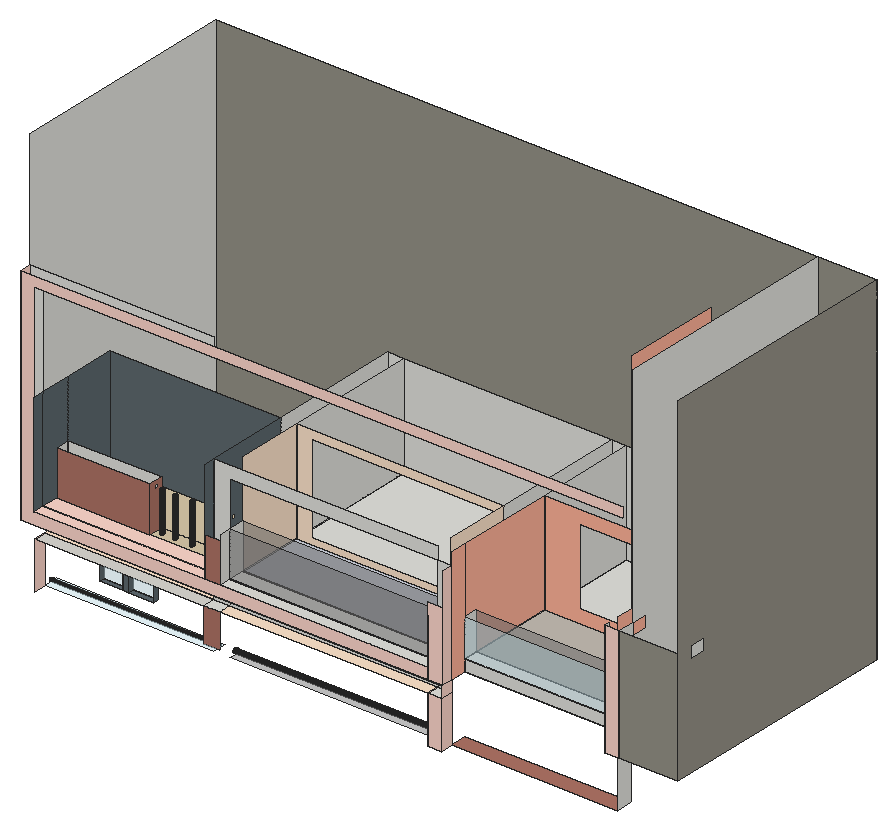
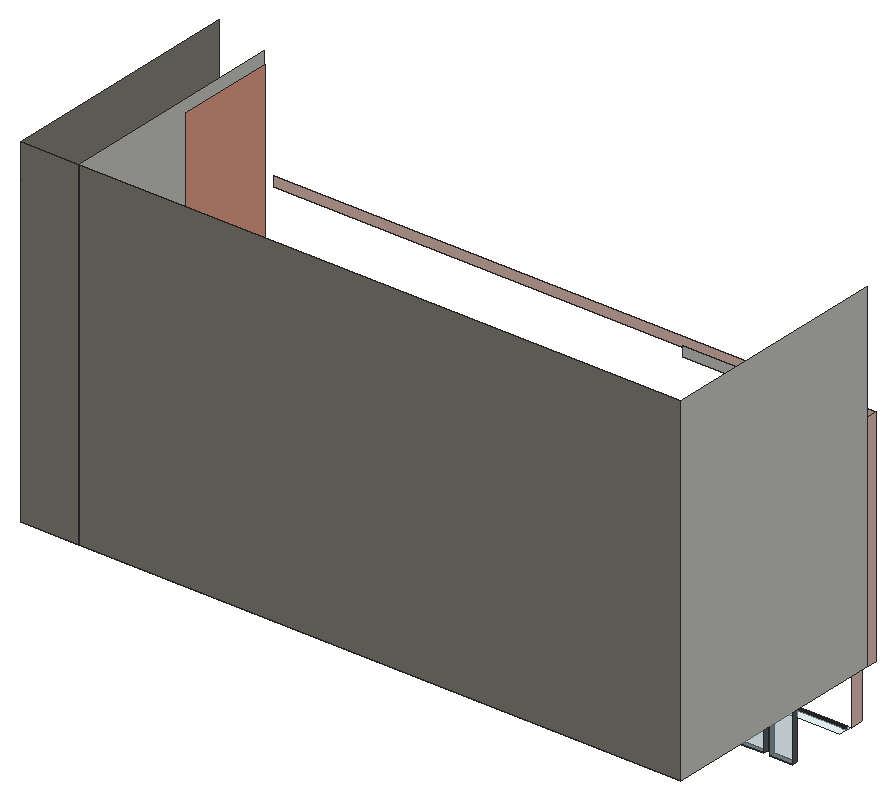
# SketchUp Ruby script. Lengths in inches.
U = 1.inch
M = Sketchup.active_model
def pt(a) = Geom::Point3d.new(a.map { |v| v * U })
def face(e, loops, mat)
  f = e.add_face(loops[0].map { |a| pt(a) })
  loops[1..].each { |l| e.add_face(l.map { |a| pt(a) }).erase! }
  f.material = f.back_material = mat if mat
  f
end
# faces: each face lists its corners as indices into pts; further lists are holes
def faces(e, pts, list, mat = nil) = list.each { |f| face(e, (f[0].is_a?(Array) ? f : [f]).map { |l| l.map { |i| pts[i] } }, mat) }
# xy, xz, yz: faces in a plane at the given z, y or x. An outline is a flat list of corners, or four numbers for a rectangle; further outlines are holes
def ring(l) = l.size == 4 ? [[l[0], l[1]], [l[2], l[1]], [l[2], l[3]], [l[0], l[3]]] : l.each_slice(2).to_a
def flat(e, list, mat, &to3) = list.each { |f| face(e, (f[0].is_a?(Array) ? f : [f]).map { |l| ring(l).map { |u, v| to3.(u, v) } }, mat) }
def xy(e, z, list, mat = nil) = flat(e, list, mat) { |x, y| [x, y, z] }
def xz(e, y, list, mat = nil) = flat(e, list, mat) { |x, z| [x, y, z] }
def yz(e, x, list, mat = nil) = flat(e, list, mat) { |y, z| [x, y, z] }
def lines(e, pts, list) = list.each { |a, b| e.add_line(pt(pts[a]), pt(pts[b])) }
# prism: a flat outline (further loops are holes) pulled along v
def prism(e, loops, v, mat = nil)
  f = face(e, loops, mat); d = Geom::Vector3d.new(v.map { |x| x * U })
  f.pushpull(f.normal.samedirection?(d) ? d.length : -d.length)
end
def box(e, o, s, mat = nil) = prism(e, [[o, [o[0] + s[0], o[1], o[2]], [o[0] + s[0], o[1] + s[1], o[2]], [o[0], o[1] + s[1], o[2]]]], [0, 0, s[2]], mat)
def at(x, y, z, deg = 0) = Geom::Transformation.translation(pt([x, y, z])) * Geom::Transformation.rotation(ORIGIN, Z_AXIS, deg.degrees)
def axes(o, x, y, z) = Geom::Transformation.new([*x, 0, *y, 0, *z, 0, *pt(o).to_a, 1])
def part(name) = M.definitions.add(name)
# library, detail: a bought-in or finely detailed component or shape, given as its bounding box
def library(name, o, s) = part(name).tap { |d| box(d.entities, o, s) }
def detail(e, o, s) = box(e.add_group.entities, o, s)
def put(e, d, t, mat = nil) = e.add_instance(d, t).tap { |i| i.material = mat if mat }
def group(e, t, mat = nil) = e.add_group.tap { |g| g.transformation = t; g.material = mat if mat }.entities
root = M.entities
M.materials.add("[Color B01]").color = [255, 216, 204]
M.materials.add("[Color B02]").color = [255, 178, 153]
M.materials.add("[Color C01]").color = [255, 229, 204]
M.materials.add("[Field Rectangle Tile]").color = [196, 189, 179]
M.materials.add("[Field Square Tile]").color = [217, 201, 169]
M.materials.add("[Formica Graystone]").color = [149, 146, 135]
M.materials.add("[Formica Laminate Dark]").color = [50, 53, 60]
M.materials.add("[Formica Speckled Grey]").color = [94, 105, 111]
M.materials.add("[Marble Carrara Floor Tile]").color = [204, 208, 219]
M.materials.add("[Stone Flagstone Ashlar]").color = [175, 116, 102]
M.materials.add("[Stone Flagstone Ashlar]1").color = [175, 116, 102]
M.materials.add("[Terrazzo Tile Light]").color = [219, 217, 210]
M.materials.add("[Translucent Glass Gray]").color = [128, 128, 128]
M.materials["[Translucent Glass Gray]"].alpha = 0.5
M.materials.add("[Translucent Glass Safety]").color = [204, 235, 244]
M.materials["[Translucent Glass Safety]"].alpha = 0.5
M.materials.add("[Wood Veneer 01]").color = [76, 44, 23]
xy(root,1199.4,[[734.47,1058.36,806.25,1074.11],[825.49,1058.36,901.24,1074.11]],"[Formica Speckled Grey]")
xy(root,1241.6875,[[1950.59,899.87,2463.34,950.43]],"[Stone Flagstone Ashlar]")
xy(root,1241.6875,[[1263.92,899.87,1905.54,941.11]],"[Translucent Glass Gray]")
xy(root,1241.6875,[[691.11,899.87,1214.63,947.14]],"[Translucent Glass Safety]")
xy(root,1376.27,[[2056.35,1110.15,2178.28,1136.84],[2208.51,1110.15,2344.68,1136.84]])
xy(root,1382.52,[[1331.05,1053.48,1447.61,1074.11],[1463.69,1053.48,1579.86,1074.11],[1595.94,1053.48,1706.36,1074.11],[1722.44,1053.48,1816.68,1074.11]],"[Wood Veneer 01]")
xy(root,1383.92,[[734.47,1058.36,806.25,1074.11],[825.49,1058.36,901.24,1074.11]],"[Formica Speckled Grey]")
xy(root,1386.6,[[927.6,1058.36,1038.4,1074.11],[1057.92,1058.36,1179.55,1074.11]],"[Formica Speckled Grey]")
xy(root,1387.1,[[1214.63,861.43,1263.92,899.87],[1905.54,861.43,1950.59,899.87]])
xy(root,1387.1,[[1263.92,861.43,1905.54,899.87],[691.11,899.87,1905.54,950.43]],"[Color C01]")
xy(root,1387.1,[[691.11,861.43,1214.63,899.87]],"[Terrazzo Tile Light]")
xy(root,1392.23,[[2040.39,1110.15,2360.64,1136.84]])
xy(root,1398.44,[[719.95,1058.36,915.76,1074.11],[915.76,1058.36,1191.39,1074.11]])
xy(root,1400.05,[[1313.52,1053.48,1834.21,1074.11]])
xy(root,1424.1875,[[2463.34,849.3125,2463.34,1136.84,1950.59,1136.84,1950.59,1571.68,1905.54,1571.68,1905.54,1074.11,1263.92,1074.11,1263.92,1571.68,1214.63,1571.68,1214.63,1074.11,691.11,1074.11,691.11,950.43,1214.63,950.43,1214.63,899.87,646.49,899.87,646.49,1616.29,2507.95,1616.29,2507.95,849.3125],[2507.95,849.3125,2688.89,1616.29],[646.49,861.43,1950.59,863.74],[646.49,863.74,1214.63,899.87],[1214.63,863.74,1263.92,899.87],
  [1263.92,863.74,1905.54,899.87],[1905.54,863.74,1950.59,899.87],[1214.63,899.87,1263.92,950.43],[1263.92,899.87,1905.54,950.43],[1905.54,899.87,1950.59,1571.68],
  [1214.63,950.43,1263.92,1571.68]])
xy(root,1424.1875,[[1950.59,950.43,2463.34,1136.84]],"[Color B02]")
xy(root,1424.1875,[[1263.92,950.43,1905.54,1074.11]],"[Color C01]")
xy(root,1424.1875,[[691.11,950.43,1214.63,1074.11]],"[Terrazzo Tile Light]")
xy(root,1460.1875,[[1214.63,863.74,1263.92,899.87],[1263.92,863.74,1905.54,899.87],[1214.63,899.87,1263.92,950.43],[1263.92,899.87,1905.54,950.43],[686.75,950.43,976.71,994.87],
  [1950.59,950.43,1950.59,992.68,2463.4,992.68,2463.34,954.56,2463.34,950.43],[994.85,967.7,993.36,967.89,991.97,968.47,990.78,969.38,989.87,970.57,989.29,971.96,989.1,973.45,989.29,974.93,989.87,976.32,990.78,977.51,991.97,978.43,993.36,979,994.85,979.2,996.34,979,997.72,978.43,998.91,977.51,999.83,976.32,1000.4,974.93,1000.6,973.45,1000.4,971.96,999.83,970.57,998.91,969.38,997.72,968.47,996.34,967.89],[1036.41,967.7,1034.92,967.89,1033.54,968.47,1032.34,969.38,1031.43,970.57,1030.86,971.96,1030.66,973.45,1030.86,974.93,1031.43,976.32,1032.34,977.51,1033.54,978.43,1034.92,979,1036.41,979.2,1037.9,979,1039.29,978.43,1040.48,977.51,1041.39,976.32,1041.96,974.93,1042.16,973.45,1041.96,971.96,1041.39,970.57,1040.48,969.38,1039.29,968.47,1037.9,967.89],[1087.54,967.7,1086.05,967.89,1084.66,968.47,1083.47,969.38,1082.56,970.57,1081.98,971.96,1081.79,973.45,1081.98,974.93,1082.56,976.32,1083.47,977.51,1084.66,978.43,1086.05,979,1087.54,979.2,1089.02,979,1090.41,978.43,1091.6,977.51,1092.51,976.32,1093.09,974.93,1093.29,973.45,1093.09,971.96,1092.51,970.57,1091.6,969.38,1090.41,968.47,1089.02,967.89],[1142.72,967.7,1141.23,967.89,1139.85,968.47,1138.66,969.38,1137.74,970.57,1137.17,971.96,1136.97,973.45,1137.17,974.93,1137.74,976.32,1138.66,977.51,1139.85,978.43,1141.23,979,1142.72,979.2,1144.21,979,1145.6,978.43,1146.79,977.51,1147.7,976.32,1148.28,974.93,1148.47,973.45,1148.28,971.96,1147.7,970.57,1146.79,969.38,1145.6,968.47,1144.21,967.89],
  [1194.79,967.7,1193.3,967.89,1191.91,968.47,1190.72,969.38,1189.81,970.57,1189.23,971.96,1189.04,973.45,1189.23,974.93,1189.81,976.32,1190.72,977.51,1191.91,978.43,1193.3,979,1194.79,979.2,1196.27,979,1197.66,978.43,1198.85,977.51,1199.76,976.32,1200.34,974.93,1200.54,973.45,1200.34,971.96,1199.76,970.57,1198.85,969.38,1197.66,968.47,1196.27,967.89],[1263.92,1156.55,1905.54,1571.68],[1950.59,1257.37,2463.8,1257.37,2464.28,1571.68,1950.59,1571.68],[2463.8,1257.37,2464.28,1571.68,2464.28,1257.37]])
xy(root,1460.1875,[[686.75,863.74,1214.63,899.87],[686.75,899.87,1214.63,950.43]],"[Color B01]")
xy(root,1460.1875,[[1950.59,992.68,2463.4,992.68,2463.8,1257.37,1950.59,1257.37]],"[Field Rectangle Tile]")
xy(root,1460.1875,[[[976.71,950.43,1214.63,994.87],[994.85,967.7,993.36,967.89,991.97,968.47,990.78,969.38,989.87,970.57,989.29,971.96,989.1,973.45,989.29,974.93,989.87,976.32,990.78,977.51,991.97,978.43,993.36,979,994.85,979.2,996.34,979,997.72,978.43,998.91,977.51,999.83,976.32,1000.4,974.93,1000.6,973.45,1000.4,971.96,999.83,970.57,998.91,969.38,997.72,968.47,996.34,967.89],[1194.79,967.7,1193.3,967.89,1191.91,968.47,1190.72,969.38,1189.81,970.57,1189.23,971.96,1189.04,973.45,1189.23,974.93,1189.81,976.32,1190.72,977.51,1191.91,978.43,1193.3,979,1194.79,979.2,1196.27,979,1197.66,978.43,1198.85,977.51,1199.76,976.32,1200.34,974.93,1200.54,973.45,1200.34,971.96,1199.76,970.57,1198.85,969.38,1197.66,968.47,1196.27,967.89],[1036.41,967.7,1034.92,967.89,1033.54,968.47,1032.34,969.38,1031.43,970.57,1030.86,971.96,1030.66,973.45,1030.86,974.93,1031.43,976.32,1032.34,977.51,1033.54,978.43,1034.92,979,1036.41,979.2,1037.9,979,1039.29,978.43,1040.48,977.51,1041.39,976.32,1041.96,974.93,1042.16,973.45,1041.96,971.96,1041.39,970.57,1040.48,969.38,1039.29,968.47,1037.9,967.89],[1142.72,967.7,1141.23,967.89,1139.85,968.47,1138.66,969.38,1137.74,970.57,1137.17,971.96,1136.97,973.45,1137.17,974.93,1137.74,976.32,1138.66,977.51,1139.85,978.43,1141.23,979,1142.72,979.2,1144.21,979,1145.6,978.43,1146.79,977.51,1147.7,976.32,1148.28,974.93,1148.47,973.45,1148.28,971.96,1147.7,970.57,1146.79,969.38,1145.6,968.47,1144.21,967.89],[1087.54,967.7,1086.05,967.89,1084.66,968.47,1083.47,969.38,1082.56,970.57,1081.98,971.96,1081.79,973.45,1081.98,974.93,1082.56,976.32,1083.47,977.51,1084.66,978.43,1086.05,979,1087.54,979.2,1089.02,979,1090.41,978.43,1091.6,977.51,1092.51,976.32,1093.09,974.93,1093.29,973.45,1093.09,971.96,1092.51,970.57,1091.6,969.38,1090.41,968.47,1089.02,967.89]],[686.75,994.87,1214.63,1156.55]],"[Field Square Tile]")
xy(root,1460.1875,[[1263.92,950.43,1905.54,1156.55]],"[Marble Carrara Floor Tile]")
xz(root,849.3125,[[2463.34,1424.1875,2507.95,1776.9375]],"[Color B01]")
xz(root,849.3125,[[2507.95,1424.1875,2688.89,1776.9375]],"[Formica Graystone]")
xz(root,861.43,[[1905.54,1241.6875,1950.59,1387.1]],"[Color B01]")
xz(root,861.43,[[1214.63,1280.46,1263.92,1387.1]],"[Stone Flagstone Ashlar]1")
xz(root,863.74,[[646.49,1424.1875,1905.54,1424.1875,1905.54,1460.1875,686.75,1460.1875,686.75,2083.5625,2507.95,2083.5625,2507.95,2114.125,646.49,2114.125],[1905.54,1424.1875,1950.59,1639.44]],"[Color B01]")
xz(root,863.74,[[1214.63,1460.1875,1263.92,1581.51]],"[Stone Flagstone Ashlar]1")
xz(root,899.87,[[1214.63,1387.1,1263.92,1424.1875],[1263.92,1387.1,1905.54,1424.1875],[1905.54,1387.1,1950.59,1424.1875],[646.49,1424.1875,646.49,2114.125,1214.63,2114.125,1214.63,2083.5625,686.75,2083.5625,686.75,1460.1875,1905.54,1460.1875,1905.54,1424.1875],[1905.54,1424.1875,1950.59,1739.53],
  [1214.63,1460.1875,1214.63,1776.9375,1905.54,1776.9375,1905.54,1739.53,1263.92,1739.53,1263.92,1460.1875]])
xz(root,899.87,[[1263.92,1460.1875,1905.54,1600.3125]],"[Translucent Glass Gray]")
xz(root,950.43,[[691.11,1387.1,1905.54,1424.1875],[1214.63,1424.1875,1263.92,1460.1875],[1263.92,1424.1875,1905.54,1460.1875],[1950.59,1424.1875,2463.34,1460.1875]])
xz(root,950.43,[[686.75,1460.1875,976.71,1600.3125]],"[Stone Flagstone Ashlar]")
xz(root,950.43,[[1263.92,1460.1875,1905.54,1600.3125]],"[Translucent Glass Gray]")
xz(root,950.43,[[1950.59,1460.1875,2463.34,1576.3125]],"[Translucent Glass Safety]")
xz(root,992.68,[[1950.59,1460.1875,2463.4,1576.3125]],"[Translucent Glass Gray]")
xz(root,994.87,[[686.75,1460.1875,976.71,1600.3125]])
xz(root,1058.36,[[806.25,1199.4,825.49,1383.92]],"[Formica Speckled Grey]")
xz(root,1074.11,[[734.47,1199.4,806.25,1383.92],[825.49,1199.4,901.24,1383.92]],"[Translucent Glass Safety]")
xz(root,1156.55,[[[1263.92,1460.1875,1905.54,1776.9375],[1311,1479.27,1873.75,1752.08]]],"[Color C01]")
xz(root,1156.55,[[686.75,1460.1875,1214.63,1776.9375]],"[Formica Speckled Grey]")
xz(root,1257.37,[[[1950.59,1460.1875,2464.28,1776.9375],[2060.83,1501.65,2333.7,1736.15]]],"[Color B02]")
xz(root,1571.68,[[1214.63,1424.1875,1263.92,1776.9375],[1905.54,1424.1875,1950.59,1776.9375],[1263.92,1460.1875,1905.54,1776.9375],[1950.59,1460.1875,2464.28,1776.9375]])
xz(root,1616.29,[[646.49,1424.1875,2507.95,2476.875],[2507.95,1424.1875,2688.89,2476.875]],"[Formica Graystone]")
yz(root,646.49,[[899.87,1424.1875,1616.29,2476.875]])
yz(root,646.49,[[863.74,1424.1875,899.87,2114.125]],"[Color B01]")
yz(root,686.75,[[950.43,1460.1875,994.87,1600.3125]])
yz(root,686.75,[[863.74,1460.1875,899.87,1776.9375],[899.87,1460.1875,950.43,1460.1875,950.43,1600.3125,994.87,1600.3125,994.87,1776.9375,899.87,1776.9375],[994.87,1460.1875,1156.55,1776.9375]],"[Formica Speckled Grey]")
yz(root,691.11,[[861.43,1241.6875,899.87,1387.1]],"[Color B01]")
yz(root,734.47,[[1058.36,1199.4,1074.11,1383.92]],"[Formica Speckled Grey]")
yz(root,806.25,[[1058.36,1199.4,1074.11,1383.92]],"[Formica Speckled Grey]")
yz(root,825.49,[[1058.36,1199.4,1074.11,1383.92]],"[Formica Speckled Grey]")
yz(root,901.24,[[1058.36,1199.4,1074.11,1383.92]],"[Formica Speckled Grey]")
yz(root,976.71,[[[950.43,1460.1875,994.87,1600.3125],[973.87,1576.82,972.15,1577.04,970.56,1577.7,969.18,1578.76,968.13,1580.13,967.47,1581.73,967.24,1583.44,967.47,1585.16,968.13,1586.75,969.18,1588.125,970.56,1589.18,972.15,1589.84,973.87,1590.07,975.58,1589.84,977.18,1589.18,978.55,1588.125,979.61,1586.75,980.27,1585.16,980.49,1583.44,980.27,1581.73,979.61,1580.13,978.55,1578.76,977.18,1577.7,975.58,1577.04]]],"[Stone Flagstone Ashlar]")
yz(root,1214.63,[[922.41,1246.62,923.375,1246.85,924.25,1247.32,924.97,1248.01,925.5,1248.85,925.78,1249.81,925.81,1250.8,925.58,1251.77,925.11,1252.65,924.42,1253.37,923.58,1253.89,922.62,1254.18,921.625,1254.21,920.66,1253.98,919.78,1253.5,919.06,1252.82,918.54,1251.97,918.25,1251.02,918.22,1250.02,918.45,1249.05,918.93,1248.18,919.61,1247.46,920.46,1246.93,921.41,1246.65],[950.43,1424.1875,1571.68,1460.1875],[1156.55,1460.1875,1571.68,1776.9375]])
yz(root,1214.63,[[863.74,1460.1875,899.87,1776.9375],[[899.87,1460.1875,1156.55,1776.9375],[973.87,1576.82,975.58,1577.04,977.18,1577.7,978.55,1578.76,979.61,1580.13,980.27,1581.73,980.49,1583.44,980.27,1585.16,979.61,1586.75,978.55,1588.125,977.18,1589.18,975.58,1589.84,973.87,1590.07,972.15,1589.84,970.56,1589.18,969.18,1588.125,968.13,1586.75,967.47,1585.16,967.24,1583.44,967.47,1581.73,968.13,1580.13,969.18,1578.76,970.56,1577.7,972.15,1577.04]]],"[Formica Speckled Grey]")
yz(root,1263.92,[[950.43,1424.1875,1571.68,1460.1875],[863.74,1460.1875,899.87,1600.3125],[899.87,1460.1875,950.43,1600.3125],[1156.55,1460.1875,1571.68,1776.9375]])
yz(root,1263.92,[[950.43,1460.1875,1156.55,1776.9375]],"[Color C01]")
yz(root,1905.54,[[918.53,1249.2,920.23,1249.42,921.8125,1250.08,923.17,1251.12,924.21,1252.48,924.87,1254.0625,925.09,1255.76,924.87,1257.46,924.21,1259.04,923.17,1260.4,921.8125,1261.45,920.23,1262.1,918.53,1262.33,916.83,1262.1,915.25,1261.45,913.89,1260.4,912.85,1259.04,912.19,1257.46,911.97,1255.76,912.19,1254.0625,912.85,1252.48,913.89,1251.12,915.25,1250.08,916.83,1249.42],[863.74,1424.1875,899.87,1460.1875],[950.43,1424.1875,1571.68,1460.1875],[863.74,1460.1875,899.87,1600.3125],[899.87,1460.1875,950.43,1600.3125],
  [1156.55,1460.1875,1571.68,1776.9375]])
yz(root,1905.54,[[861.43,1241.6875,899.87,1387.1]],"[Color B01]")
yz(root,1905.54,[[950.43,1460.1875,1156.55,1776.9375]],"[Color C01]")
yz(root,1950.59,[[950.43,1424.1875,1571.68,1460.1875],[950.43,1460.1875,992.68,1576.3125],[1257.37,1460.1875,1571.68,1776.9375]])
yz(root,1950.59,[[861.43,1241.6875,899.87,1387.1],[861.43,1387.1,899.87,1424.1875],[863.74,1424.1875,899.87,1739.53]],"[Color B01]")
yz(root,1950.59,[[899.87,1424.1875,950.43,1776.9375],[992.68,1460.1875,1257.37,1460.1875,1257.37,1776.9375,950.43,1776.9375,950.43,1576.3125,992.68,1576.3125]],"[Color B02]")
yz(root,2463.34,[[899.87,1241.6875,950.43,1424.1875],[849.3125,1424.1875,849.3125,1776.9375,863.74,1776.9375,863.74,1739.53,899.87,1739.53,899.87,1424.1875],[950.43,1424.1875,954.56,1460.1875],[950.43,1460.1875,954.56,1576.3125]])
yz(root,2463.34,[[899.87,1424.1875,899.87,1776.9375,954.56,1776.9375,954.56,1576.3125,950.43,1576.3125,950.43,1424.1875]],"[Color B02]")
yz(root,2464.28,[[1257.37,1460.1875,1571.68,1776.9375]])
yz(root,2507.95,[[849.3125,1424.1875,849.3125,1776.9375,899.87,1776.9375,899.87,1739.53,950.43,1739.53,950.43,1776.9375,899.87,1776.9375,899.87,2476.875,1616.29,2476.875,1616.29,1424.1875]])
yz(root,2688.89,[[849.3125,1424.1875,1616.29,1424.1875,1616.29,2476.875,849.3125,2476.875,849.3125,1776.9375,950.43,1776.9375,950.43,1739.53,899.87,1739.53,899.87,1776.9375,849.3125,1776.9375]],"[Formica Graystone]")
p = [[1214.63,921.41,1246.65],[1214.63,920.46,1246.93],[691.11,920.46,1246.93],[691.11,921.41,1246.65],[1214.63,922.41,1246.62],[691.11,922.41,1246.62],
  [1214.63,923.375,1246.85],[691.11,923.375,1246.85],[1214.63,919.61,1247.46],[691.11,919.61,1247.46],[1214.63,924.25,1247.32],[691.11,924.25,1247.32],
  [1214.63,924.97,1248.01],[691.11,924.97,1248.01],[1214.63,918.93,1248.18],[691.11,918.93,1248.18],[1214.63,925.5,1248.85],[691.11,925.5,1248.85],
  [1214.63,918.45,1249.05],[691.11,918.45,1249.05],[1214.63,925.78,1249.81],[691.11,925.78,1249.81],[1214.63,918.22,1250.02],[691.11,918.22,1250.02],
  [1905.54,918.53,1249.2],[1905.54,916.83,1249.42],[1263.92,916.83,1249.42],[1263.92,918.53,1249.2],[1905.54,920.23,1249.42],[1263.92,920.23,1249.42],
  [1905.54,915.25,1250.08],[1263.92,915.25,1250.08],[1905.54,921.8125,1250.08],[1263.92,921.8125,1250.08],[1214.63,925.81,1250.8],[691.11,925.81,1250.8],
  [1214.63,918.25,1251.02],[691.11,918.25,1251.02],[1905.54,913.89,1251.12],[1263.92,913.89,1251.12],[1905.54,923.17,1251.12],[1263.92,923.17,1251.12],
  [1214.63,925.58,1251.77],[691.11,925.58,1251.77],[1214.63,918.54,1251.97],[691.11,918.54,1251.97],[1905.54,912.85,1252.48],[1263.92,912.85,1252.48],
  [1905.54,924.21,1252.48],[1263.92,924.21,1252.48],[1214.63,925.11,1252.65],[691.11,925.11,1252.65],[1214.63,919.06,1252.82],[691.11,919.06,1252.82],
  [1905.54,912.19,1254.0625],[1263.92,912.19,1254.0625],[1905.54,924.87,1254.0625],[1263.92,924.87,1254.0625],[1214.63,924.42,1253.37],[691.11,924.42,1253.37],
  [1214.63,919.78,1253.5],[691.11,919.78,1253.5],[1214.63,923.58,1253.89],[691.11,923.58,1253.89],[1214.63,920.66,1253.98],[691.11,920.66,1253.98],
  [1214.63,922.62,1254.18],[691.11,922.62,1254.18],[1214.63,921.625,1254.21],[691.11,921.625,1254.21],[1905.54,911.97,1255.76],[1263.92,911.97,1255.76],
  [1905.54,925.09,1255.76],[1263.92,925.09,1255.76],[1905.54,912.19,1257.46],[1263.92,912.19,1257.46],[1905.54,924.87,1257.46],[1263.92,924.87,1257.46],
  [1905.54,912.85,1259.04],[1263.92,912.85,1259.04],[1905.54,924.21,1259.04],[1263.92,924.21,1259.04],[1905.54,913.89,1260.4],[1263.92,913.89,1260.4],
  [1905.54,923.17,1260.4],[1263.92,923.17,1260.4],[1905.54,915.25,1261.45],[1263.92,915.25,1261.45],[1905.54,921.8125,1261.45],[1263.92,921.8125,1261.45],
  [1905.54,916.83,1262.1],[1263.92,916.83,1262.1],[1905.54,920.23,1262.1],[1263.92,920.23,1262.1],[1905.54,918.53,1262.33],[1263.92,918.53,1262.33],
  [2463.4,992.68,1460.1875],[2463.34,954.56,1460.1875],[2463.34,954.56,1576.3125],[2463.4,992.68,1576.3125],[2464.28,1571.68,1460.1875],[2463.8,1257.37,1460.1875],
  [2463.34,954.56,1776.9375],[2463.34,954.56,1788.9375],[2463.34,954.56,1923.4375],[2463.34,954.56,2114.125],[2463.34,954.56,2126.125],[2463.34,954.56,2369.6875],
  [2463.34,954.56,2379.45],[2463.34,954.56,2381.6875],[2463.34,954.56,2400.95],[2463.34,954.56,2428.82],[2463.34,954.56,2476.875],[2463.77,1237.41,2476.875],
  [2463.8,1257.37,2476.875],[2463.8,1257.37,1776.9375],[2464.28,1571.68,1776.9375],[2463.35,962.98,1592.2],[2463.36,963.19,1590.63],[2463.36,963.8,1589.17],
  [2463.36,964.76,1587.92],[2463.36,966.01,1586.95],[2463.36,967.48,1586.35],[2463.36,969.05,1586.14],[2463.37,970.61,1586.35],[2463.37,972.08,1586.95],
  [2463.37,973.33,1587.92],[2463.37,974.3,1589.17],[2463.375,974.9,1590.63],[2463.375,975.11,1592.2],[2463.375,974.9,1593.77],[2463.37,974.3,1595.23],
  [2463.37,973.33,1596.49],[2463.37,972.08,1597.45],[2463.37,970.61,1598.06],[2463.36,969.05,1598.27],[2463.36,967.48,1598.06],[2463.36,966.01,1597.45],
  [2463.36,964.76,1596.49],[2463.36,963.8,1595.23],[2463.36,963.19,1593.77],[993.36,967.89,1460.1875],[994.85,967.7,1460.1875],[994.85,967.7,1582.8125],
  [993.36,967.89,1582.8125],[996.34,967.89,1460.1875],[996.34,967.89,1582.8125],[1034.92,967.89,1460.1875],[1036.41,967.7,1460.1875],[1036.41,967.7,1581.3125],
  [1034.92,967.89,1581.3125],[1037.9,967.89,1460.1875],[1037.9,967.89,1581.3125],[1086.05,967.89,1460.1875],[1087.54,967.7,1460.1875],[1087.54,967.7,1582.25],
  [1086.05,967.89,1582.25],[1089.02,967.89,1460.1875],[1089.02,967.89,1582.25],[1141.23,967.89,1460.1875],[1142.72,967.7,1460.1875],[1142.72,967.7,1582.375],
  [1141.23,967.89,1582.375],[1144.21,967.89,1460.1875],[1144.21,967.89,1582.375],[1193.3,967.89,1460.1875],[1194.79,967.7,1460.1875],[1194.79,967.7,1583.0625],
  [1193.3,967.89,1583.0625],[1196.27,967.89,1460.1875],[1196.27,967.89,1583.0625],[991.97,968.47,1460.1875],[991.97,968.47,1582.8125],[997.72,968.47,1460.1875],
  [997.72,968.47,1582.8125],[1033.54,968.47,1460.1875],[1033.54,968.47,1581.3125],[1039.29,968.47,1460.1875],[1039.29,968.47,1581.3125],[1084.66,968.47,1460.1875],
  [1084.66,968.47,1582.25],[1090.41,968.47,1460.1875],[1090.41,968.47,1582.25],[1139.85,968.47,1460.1875],[1139.85,968.47,1582.375],[1145.6,968.47,1460.1875],
  [1145.6,968.47,1582.375],[1191.91,968.47,1460.1875],[1191.91,968.47,1583.0625],[1197.66,968.47,1460.1875],[1197.66,968.47,1583.0625],[990.78,969.38,1460.1875],
  [990.78,969.38,1582.8125],[998.91,969.38,1460.1875],[998.91,969.38,1582.8125],[1032.34,969.38,1460.1875],[1032.34,969.38,1581.3125],[1040.48,969.38,1460.1875],
  [1040.48,969.38,1581.3125],[1083.47,969.38,1460.1875],[1083.47,969.38,1582.25],[1091.6,969.38,1460.1875],[1091.6,969.38,1582.25],[1138.66,969.38,1460.1875],
  [1138.66,969.38,1582.375],[1146.79,969.38,1460.1875],[1146.79,969.38,1582.375],[1190.72,969.38,1460.1875],[1190.72,969.38,1583.0625],[1198.85,969.38,1460.1875],
  [1198.85,969.38,1583.0625],[989.87,970.57,1460.1875],[989.87,970.57,1582.8125],[999.83,970.57,1460.1875],[999.83,970.57,1582.8125],[1031.43,970.57,1460.1875],
  [1031.43,970.57,1581.3125],[1041.39,970.57,1460.1875],[1041.39,970.57,1581.3125],[1082.56,970.57,1460.1875],[1082.56,970.57,1582.25],[1092.51,970.57,1460.1875],
  [1092.51,970.57,1582.25],[1137.74,970.57,1460.1875],[1137.74,970.57,1582.375],[1147.7,970.57,1460.1875],[1147.7,970.57,1582.375],[1189.81,970.57,1460.1875],
  [1189.81,970.57,1583.0625],[1199.76,970.57,1460.1875],[1199.76,970.57,1583.0625],[989.29,971.96,1460.1875],[989.29,971.96,1582.8125],[1000.4,971.96,1460.1875],
  [1000.4,971.96,1582.8125],[1030.86,971.96,1460.1875],[1030.86,971.96,1581.3125],[1041.96,971.96,1460.1875],[1041.96,971.96,1581.3125],[1081.98,971.96,1460.1875],
  [1081.98,971.96,1582.25],[1093.09,971.96,1460.1875],[1093.09,971.96,1582.25],[1137.17,971.96,1460.1875],[1137.17,971.96,1582.375],[1148.28,971.96,1460.1875],
  [1148.28,971.96,1582.375],[1189.23,971.96,1460.1875],[1189.23,971.96,1583.0625],[1200.34,971.96,1460.1875],[1200.34,971.96,1583.0625],[989.1,973.45,1460.1875],
  [989.1,973.45,1582.8125],[1000.6,973.45,1460.1875],[1000.6,973.45,1582.8125],[1030.66,973.45,1460.1875],[1030.66,973.45,1581.3125],[1042.16,973.45,1460.1875],
  [1042.16,973.45,1581.3125],[1081.79,973.45,1460.1875],[1081.79,973.45,1582.25],[1093.29,973.45,1460.1875],[1093.29,973.45,1582.25],[1136.97,973.45,1460.1875],
  [1136.97,973.45,1582.375],[1148.47,973.45,1460.1875],[1148.47,973.45,1582.375],[1189.04,973.45,1460.1875],[1189.04,973.45,1583.0625],[1200.54,973.45,1460.1875],
  [1200.54,973.45,1583.0625],[989.29,974.93,1460.1875],[989.29,974.93,1582.8125],[1000.4,974.93,1460.1875],[1000.4,974.93,1582.8125],[1030.86,974.93,1460.1875],
  [1030.86,974.93,1581.3125],[1041.96,974.93,1460.1875],[1041.96,974.93,1581.3125],[1081.98,974.93,1460.1875],[1081.98,974.93,1582.25],[1093.09,974.93,1460.1875],
  [1093.09,974.93,1582.25],[1137.17,974.93,1460.1875],[1137.17,974.93,1582.375],[1148.28,974.93,1460.1875],[1148.28,974.93,1582.375],[1189.23,974.93,1460.1875],
  [1189.23,974.93,1583.0625],[1200.34,974.93,1460.1875],[1200.34,974.93,1583.0625],[989.87,976.32,1460.1875],[989.87,976.32,1582.8125],[999.83,976.32,1460.1875],
  [999.83,976.32,1582.8125],[1031.43,976.32,1460.1875],[1031.43,976.32,1581.3125],[1041.39,976.32,1460.1875],[1041.39,976.32,1581.3125],[1082.56,976.32,1460.1875],
  [1082.56,976.32,1582.25],[1092.51,976.32,1460.1875],[1092.51,976.32,1582.25],[1137.74,976.32,1460.1875],[1137.74,976.32,1582.375],[1147.7,976.32,1460.1875],
  [1147.7,976.32,1582.375],[1189.81,976.32,1460.1875],[1189.81,976.32,1583.0625],[1199.76,976.32,1460.1875],[1199.76,976.32,1583.0625],[990.78,977.51,1460.1875],
  [990.78,977.51,1582.8125],[998.91,977.51,1460.1875],[998.91,977.51,1582.8125],[1032.34,977.51,1460.1875],[1032.34,977.51,1581.3125],[1040.48,977.51,1460.1875],
  [1040.48,977.51,1581.3125],[1083.47,977.51,1460.1875],[1083.47,977.51,1582.25],[1091.6,977.51,1460.1875],[1091.6,977.51,1582.25],[1138.66,977.51,1460.1875],
  [1138.66,977.51,1582.375],[1146.79,977.51,1460.1875],[1146.79,977.51,1582.375],[1190.72,977.51,1460.1875],[1190.72,977.51,1583.0625],[1198.85,977.51,1460.1875],
  [1198.85,977.51,1583.0625],[991.97,978.43,1460.1875],[991.97,978.43,1582.8125],[997.72,978.43,1460.1875],[997.72,978.43,1582.8125],[1033.54,978.43,1460.1875],
  [1033.54,978.43,1581.3125],[1039.29,978.43,1460.1875],[1039.29,978.43,1581.3125],[1084.66,978.43,1460.1875],[1084.66,978.43,1582.25],[1090.41,978.43,1460.1875],
  [1090.41,978.43,1582.25],[1139.85,978.43,1460.1875],[1139.85,978.43,1582.375],[1145.6,978.43,1460.1875],[1145.6,978.43,1582.375],[1191.91,978.43,1460.1875],
  [1191.91,978.43,1583.0625],[1197.66,978.43,1460.1875],[1197.66,978.43,1583.0625],[993.36,979,1460.1875],[993.36,979,1582.8125],[996.34,979,1460.1875],
  [996.34,979,1582.8125],[1034.92,979,1460.1875],[1034.92,979,1581.3125],[1037.9,979,1460.1875],[1037.9,979,1581.3125],[1086.05,979,1460.1875],
  [1086.05,979,1582.25],[1089.02,979,1460.1875],[1089.02,979,1582.25],[1141.23,979,1460.1875],[1141.23,979,1582.375],[1144.21,979,1460.1875],
  [1144.21,979,1582.375],[1193.3,979,1460.1875],[1193.3,979,1583.0625],[1196.27,979,1460.1875],[1196.27,979,1583.0625],[994.85,979.2,1460.1875],
  [994.85,979.2,1582.8125],[1036.41,979.2,1460.1875],[1036.41,979.2,1581.3125],[1087.54,979.2,1460.1875],[1087.54,979.2,1582.25],[1142.72,979.2,1460.1875],
  [1142.72,979.2,1582.375],[1194.79,979.2,1460.1875],[1194.79,979.2,1583.0625],[2463.34,1012.29,1424.1875],[2463.34,1012.29,1460.1875],[2463.34,983.36,1424.1875],
  [2463.34,983.36,1460.1875]]
faces(root,p,[[0,1,2,3],[4,0,3,5],[6,4,5,7],[1,8,9,2],[10,6,7,11],[12,10,11,13],[8,14,15,9],[16,12,13,17],
  [14,18,19,15],[20,16,17,21],[18,22,23,19],[24,25,26,27],[28,24,27,29],[25,30,31,26],[32,28,29,33],[34,20,21,35],
  [22,36,37,23],[30,38,39,31],[40,32,33,41],[42,34,35,43],[36,44,45,37],[38,46,47,39],[48,40,41,49],[50,42,43,51],
  [44,52,53,45],[46,54,55,47],[56,48,49,57],[58,50,51,59],[52,60,61,53],[62,58,59,63],[60,64,65,61],[66,62,63,67],
  [64,68,69,65],[54,70,71,55],[72,56,57,73],[68,66,67,69],[70,74,75,71],[76,72,73,77],[74,78,79,75],[80,76,77,81],
  [78,82,83,79],[84,80,81,85],[82,86,87,83],[88,84,85,89],[86,90,91,87],[92,88,89,93],[90,94,95,91],[94,92,93,95]],"[Formica Laminate Dark]")
faces(root,p,[[96,97,98,99]])
faces(root,p,[[[100,101,96,99,98,102,103,104,105,106,107,108,109,110,111,112,113,114,115,116],[117,118,119,120,121,122,123,124,125,126,127,128,129,130,131,132,133,134,135,136,137,138,139,140]]],"[Color B02]")
faces(root,p,[[141,142,143,144],[142,145,146,143],[147,148,149,150],[148,151,152,149],[153,154,155,156],[154,157,158,155],[159,160,161,162],[160,163,164,161],
  [165,166,167,168],[166,169,170,167],[171,141,144,172],[145,173,174,146],[175,147,150,176],[151,177,178,152],[179,153,156,180],[157,181,182,158],
  [183,159,162,184],[163,185,186,164],[187,165,168,188],[169,189,190,170],[191,171,172,192],[173,193,194,174],[195,175,176,196],[177,197,198,178],
  [199,179,180,200],[181,201,202,182],[203,183,184,204],[185,205,206,186],[207,187,188,208],[189,209,210,190],[211,191,192,212],[193,213,214,194],
  [215,195,196,216],[197,217,218,198],[219,199,200,220],[201,221,222,202],[223,203,204,224],[205,225,226,206],[227,207,208,228],[209,229,230,210],
  [231,211,212,232],[213,233,234,214],[235,215,216,236],[217,237,238,218],[239,219,220,240],[221,241,242,222],[243,223,224,244],[225,245,246,226],
  [247,227,228,248],[229,249,250,230],[251,231,232,252],[233,253,254,234],[255,235,236,256],[237,257,258,238],[259,239,240,260],[241,261,262,242],
  [263,243,244,264],[245,265,266,246],[267,247,248,268],[249,269,270,250],[271,251,252,272],[253,273,274,254],[275,255,256,276],[257,277,278,258],
  [279,259,260,280],[261,281,282,262],[283,263,264,284],[265,285,286,266],[287,267,268,288],[269,289,290,270],[291,271,272,292],[273,293,294,274],
  [295,275,276,296],[277,297,298,278],[299,279,280,300],[281,301,302,282],[303,283,284,304],[285,305,306,286],[307,287,288,308],[289,309,310,290],
  [311,291,292,312],[293,313,314,294],[315,295,296,316],[297,317,318,298],[319,299,300,320],[301,321,322,302],[323,303,304,324],[305,325,326,306],
  [327,307,308,328],[309,329,330,310],[331,311,312,332],[313,333,334,314],[335,315,316,336],[317,337,338,318],[339,319,320,340],[321,341,342,322],
  [343,323,324,344],[325,345,346,326],[347,327,328,348],[329,349,350,330],[351,331,332,352],[333,353,354,334],[355,335,336,356],[337,357,358,338],
  [359,339,340,360],[341,361,362,342],[363,343,344,364],[345,365,366,346],[367,347,348,368],[349,369,370,350],[371,351,352,372],[353,371,372,354],
  [373,355,356,374],[357,373,374,358],[375,359,360,376],[361,375,376,362],[377,363,364,378],[365,377,378,366],[379,367,368,380],[369,379,380,370]],"[Formica Graystone]")
lines(root,p,[[381,382],[383,384]])
